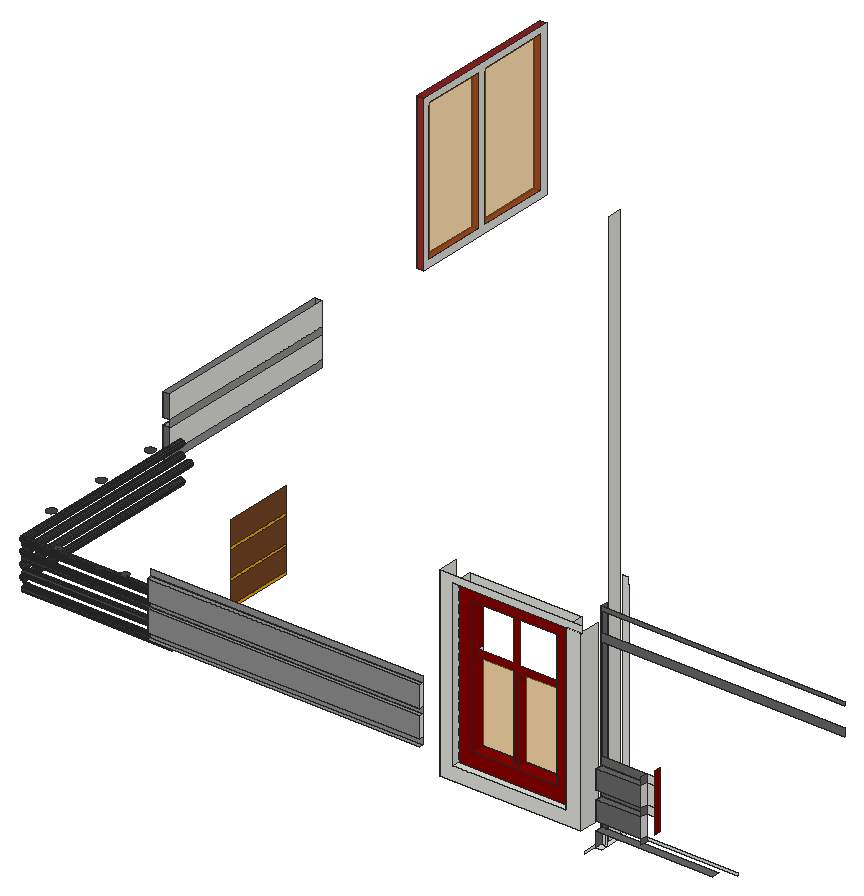
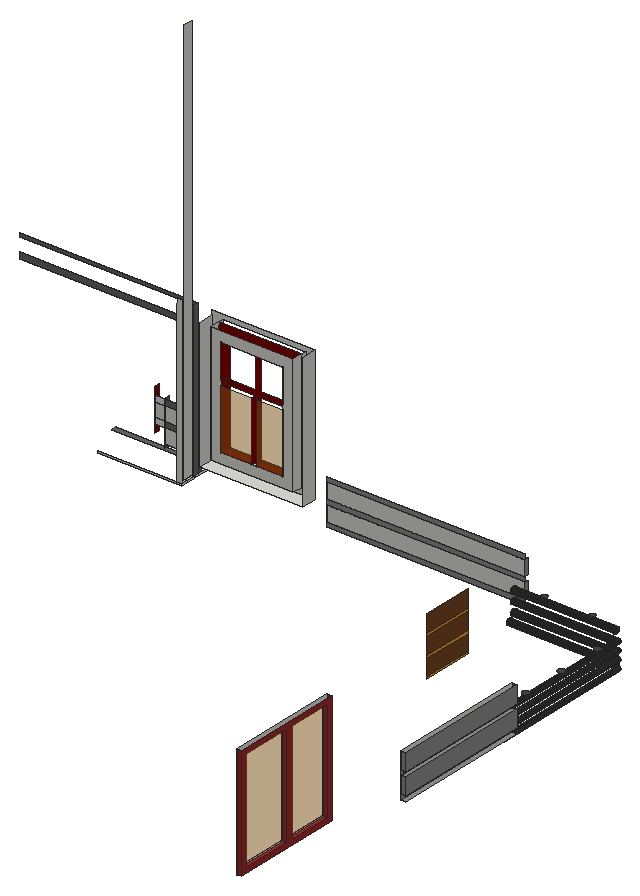
# SketchUp Ruby script. Lengths in inches.
U = 1.inch
M = Sketchup.active_model
def pt(a) = Geom::Point3d.new(a.map { |v| v * U })
def face(e, loops, mat)
  f = e.add_face(loops[0].map { |a| pt(a) })
  loops[1..].each { |l| e.add_face(l.map { |a| pt(a) }).erase! }
  f.material = f.back_material = mat if mat
  f
end
# faces: each face lists its corners as indices into pts; further lists are holes
def faces(e, pts, list, mat = nil) = list.each { |f| face(e, (f[0].is_a?(Array) ? f : [f]).map { |l| l.map { |i| pts[i] } }, mat) }
# xy, xz, yz: faces in a plane at the given z, y or x. An outline is a flat list of corners, or four numbers for a rectangle; further outlines are holes
def ring(l) = l.size == 4 ? [[l[0], l[1]], [l[2], l[1]], [l[2], l[3]], [l[0], l[3]]] : l.each_slice(2).to_a
def flat(e, list, mat, &to3) = list.each { |f| face(e, (f[0].is_a?(Array) ? f : [f]).map { |l| ring(l).map { |u, v| to3.(u, v) } }, mat) }
def xy(e, z, list, mat = nil) = flat(e, list, mat) { |x, y| [x, y, z] }
def xz(e, y, list, mat = nil) = flat(e, list, mat) { |x, z| [x, y, z] }
def yz(e, x, list, mat = nil) = flat(e, list, mat) { |y, z| [x, y, z] }
def lines(e, pts, list) = list.each { |a, b| e.add_line(pt(pts[a]), pt(pts[b])) }
# prism: a flat outline (further loops are holes) pulled along v
def prism(e, loops, v, mat = nil)
  f = face(e, loops, mat); d = Geom::Vector3d.new(v.map { |x| x * U })
  f.pushpull(f.normal.samedirection?(d) ? d.length : -d.length)
end
def box(e, o, s, mat = nil) = prism(e, [[o, [o[0] + s[0], o[1], o[2]], [o[0] + s[0], o[1] + s[1], o[2]], [o[0], o[1] + s[1], o[2]]]], [0, 0, s[2]], mat)
def at(x, y, z, deg = 0) = Geom::Transformation.translation(pt([x, y, z])) * Geom::Transformation.rotation(ORIGIN, Z_AXIS, deg.degrees)
def axes(o, x, y, z) = Geom::Transformation.new([*x, 0, *y, 0, *z, 0, *pt(o).to_a, 1])
def part(name) = M.definitions.add(name)
# library, detail: a bought-in or finely detailed component or shape, given as its bounding box
def library(name, o, s) = part(name).tap { |d| box(d.entities, o, s) }
def detail(e, o, s) = box(e.add_group.entities, o, s)
def put(e, d, t, mat = nil) = e.add_instance(d, t).tap { |i| i.material = mat if mat }
def group(e, t, mat = nil) = e.add_group.tap { |g| g.transformation = t; g.material = mat if mat }.entities
root = M.entities
M.materials.add("[0018_Brown]").color = [165, 42, 42]
M.materials.add("[0021_DarkRed]").color = [139, 0, 0]
M.materials.add("[0038_Orange]").color = [255, 165, 0]
M.materials.add("[0134_DimGray]").color = [105, 105, 105]
M.materials.add("[0137_Black]").color = [71, 71, 71]
M.materials.add("[Color M05]").color = [145, 145, 145]
M.materials.add("[Translucent Glass Gray]").color = [191, 123, 24]
M.materials["[Translucent Glass Gray]"].alpha = 0.5
M.materials.add("[Wood Veneer 01]").color = [120, 70, 37]
xy(root,135.98,[[284.66,7.0625,286.99,10.0625],[284.41,10.0625,286.99,22.0625]])
xy(root,137.03,[[284.41,10.0625,284.66,12.1875],[284.41,12.1875,284.66,13.0625],[284.66,12.1875,284.66,13.0625,284.41,13.0625,284.41,18.1875,285.29,18.1875,285.29,12.1875],[285.29,12.1875,286.17,18.1875],[284.41,18.1875,285.29,22.0625],
  [285.29,18.1875,286.17,22.0625]])
xy(root,141.65,[[82.85,16.375,200.79,18.1875]],"[Color M05]")
xy(root,142.03,[[8.875,116.75,11.875,199.5]],"[Color M05]")
xy(root,142.6875,[[284.66,7.0625,335.53,10.0625]],"[0134_DimGray]")
xy(root,142.96,[[219.91,3.1875,281.16,12.1875]])
xy(root,144.55,[[82.85,16.375,200.79,18.1875]])
xy(root,145.07,[[8.875,116.75,11.875,199.5]],"[Color M05]")
xy(root,146.27,[[284.66,7.0625,304.13,10.0625]],"[0134_DimGray]")
xy(root,148.83,[[225.66,3.1875,274.54,6.1875],[225.66,6.1875,274.54,12.1875]])
xy(root,153.65,[[82.85,16.375,200.79,18.1875]],"[Color M05]")
xy(root,154.6875,[[284.66,7.0625,304.13,10.0625]],"[0134_DimGray]")
xy(root,154.6875,[[15.96,45.8,16.47,45.87,16.93,46.06,17.33,46.37,17.64,46.77,17.84,47.24,17.9,47.74,17.84,48.24,17.64,48.71,17.33,49.11,16.93,49.41,16.47,49.61,15.96,49.67,15.46,49.61,15,49.41,14.59,49.11,14.29,48.71,14.09,48.24,14.03,47.74,14.09,47.24,14.29,46.77,14.59,46.37,15,46.06,15.46,45.87],[15.96,72.86,16.47,72.93,16.93,73.12,17.33,73.43,17.64,73.83,17.84,74.3,17.9,74.8,17.84,75.3,17.64,75.77,17.33,76.17,16.93,76.48,16.47,76.67,15.96,76.74,15.46,76.67,15,76.48,14.59,76.17,14.29,75.77,14.09,75.3,14.03,74.8,14.09,74.3,14.29,73.83,14.59,73.43,15,73.12,15.46,72.93]],"[0137_Black]")
xy(root,154.75,[[15.96,99.36,16.47,99.43,16.93,99.62,17.33,99.93,17.64,100.33,17.84,100.8,17.9,101.3,17.84,101.8,17.64,102.27,17.33,102.67,16.93,102.98,16.47,103.17,15.96,103.24,15.46,103.17,15,102.98,14.59,102.67,14.29,102.27,14.09,101.8,14.03,101.3,14.09,100.8,14.29,100.33,14.59,99.93,15,99.62,15.46,99.43]],"[0137_Black]")
xy(root,154.83,[[247.4,9.1875,250.1,12.1875]])
xy(root,154.83,[[231.66,6.1875,268.54,6.1875,268.54,12.1875,250.1,12.1875,250.1,9.1875,247.4,9.1875,247.4,12.1875,231.66,12.1875]],"[0021_DarkRed]")
xy(root,155.15,[[8.875,116.75,11.875,199.5]],"[Color M05]")
xy(root,155.78,[[8.875,254.47,11.875,321.35]],"[0018_Brown]")
xy(root,156.3125,[[35.53,25.16,35.9375,25.1875,36.32,25.32,36.66,25.54,36.93,25.85,37.11,26.21,37.2,26.61,37.17,27.02,37.04,27.41,36.82,27.75,36.51,28.02,36.15,28.2,35.75,28.28,35.34,28.25,34.95,28.125,34.61,27.9,34.34,27.59,34.16,27.23,34.08,26.83,34.1,26.42,34.23,26.04,34.46,25.7,34.76,25.43,35.13,25.24],[64.53,25.16,64.9375,25.1875,65.32,25.32,65.66,25.54,65.93,25.85,66.11,26.21,66.2,26.61,66.17,27.02,66.04,27.41,65.82,27.75,65.51,28.02,65.15,28.2,64.75,28.28,64.34,28.25,63.95,28.125,63.61,27.9,63.34,27.59,63.16,27.23,63.08,26.83,63.1,26.42,63.23,26.04,63.46,25.7,63.76,25.43,64.13,25.24]],"[0137_Black]")
xy(root,156.55,[[82.85,16.375,200.79,18.1875]])
xy(root,158.19,[[8.875,116.75,11.875,199.5]],"[Color M05]")
xy(root,158.27,[[284.66,7.0625,304.13,10.0625]],"[0134_DimGray]")
xy(root,158.78,[[8.875,257.47,11.875,284.27],[8.875,287.91,11.875,318.35]],"[0018_Brown]")
xy(root,165.65,[[82.85,16.375,200.79,18.1875]],"[Color M05]")
xy(root,166.6875,[[284.66,7.0625,304.13,10.0625]],"[0134_DimGray]")
xz(root,3.1875,[[219.91,142.96,281.16,142.96,281.16,219.83,274.54,219.83,274.54,148.83,225.66,148.83,225.66,219.83,281.47,219.83,281.47,222.71,219.91,222.71]])
xz(root,6.1875,[[[225.66,148.83,274.54,219.83],[231.66,154.83,268.54,213.83]]],"[0021_DarkRed]")
xz(root,7.0625,[[284.66,146.27,304.13,154.6875],[284.66,158.27,304.13,166.6875]],"[0134_DimGray]")
xz(root,9.1875,[[247.4,154.83,250.1,154.83,250.1,190.54,268.54,190.54,268.54,193.6,250.1,193.6,250.1,213.83,247.4,213.83,247.4,193.6,231.66,193.6,231.66,190.54,247.4,190.54]],"[0021_DarkRed]")
xz(root,10.0625,[[284.41,135.98,284.66,137.03],[284.66,135.98,286.17,142.6875],[286.17,135.98,286.99,142.6875],[284.66,146.27,286.17,154.6875],[286.17,146.27,286.99,154.6875],
  [286.99,146.27,304.13,154.6875],[304.13,154.6875,310.13,158.27],[284.66,158.27,286.17,166.6875],[286.17,158.27,286.99,166.6875],[286.99,158.27,304.13,166.6875],
  [304.13,158.27,310.13,166.6875],[304.13,166.6875,310.13,170.27]])
xz(root,10.0625,[[284.41,137.03,284.66,137.03,284.66,214.6875,390.0625,214.6875,390.0625,218.27,284.66,218.27,284.66,226.6875,390.0625,226.6875,390.0625,228.47,284.41,228.47],[284.66,154.6875,304.13,158.27],[284.66,166.6875,304.13,170.27]],"[0134_DimGray]")
xz(root,12.1875,[[[225.66,148.83,274.54,219.83],[231.66,154.83,268.54,213.83]]])
xz(root,12.1875,[[231.66,154.83,247.4,190.54],[250.1,154.83,268.54,190.54]],"[Translucent Glass Gray]")
xz(root,13.0625,[[284.41,137.03,284.66,228.47]])
xz(root,16.375,[[82.85,144.55,200.79,153.65],[82.85,156.55,200.79,165.65]],"[Color M05]")
xz(root,18.1875,[[82.85,144.55,200.79,153.65],[82.85,156.55,200.79,165.65]])
xz(root,18.1875,[[82.85,141.65,200.79,144.55],[82.85,153.65,200.79,156.55],[82.85,165.65,200.79,168.55]],"[Color M05]")
xz(root,22.0625,[[284.41,135.98,286.99,137.03],[286.99,135.98,334.1,137.03],[284.41,137.03,286.99,137.03,286.99,232.22,286.52,232.22,286.52,235.42,284.41,235.42]])
xz(root,116.75,[[8.875,145.07,11.875,155.15],[8.875,158.19,11.875,168.28]],"[0134_DimGray]")
xz(root,121.3125,[[17.02,139.87,16.66,139.91,16.33,140.05,16.05,140.27,15.83,140.55,15.69,140.89,15.65,141.24,15.69,141.6,15.83,141.93,16.05,142.21,16.33,142.43,16.66,142.57,17.02,142.62,17.375,142.57,17.71,142.43,17.99,142.21,18.21,141.93,18.35,141.6,18.4,141.24,18.35,140.89,18.21,140.55,17.99,140.27,17.71,140.05,17.375,139.91]])
xz(root,199.5,[[8.875,145.07,11.875,155.15],[8.875,158.19,11.875,168.28]],"[Color M05]")
xz(root,254.47,[[8.875,155.78,11.875,222.65]],"[0018_Brown]")
xz(root,257.47,[[8.875,158.78,11.875,219.65]],"[0018_Brown]")
xz(root,284.27,[[8.875,158.78,11.875,219.65]],"[0018_Brown]")
xz(root,287.91,[[8.875,158.78,11.875,219.65]],"[0018_Brown]")
xz(root,318.35,[[8.875,158.78,11.875,219.65]],"[0018_Brown]")
xz(root,321.35,[[8.875,155.78,11.875,222.65]],"[0018_Brown]")
yz(root,8.875,[[[254.47,155.78,321.35,222.65],[287.91,158.78,318.35,219.65],[257.47,158.78,284.27,219.65]]],"[0018_Brown]")
yz(root,8.875,[[116.75,145.07,199.5,155.15],[116.75,158.19,199.5,168.28]],"[Color M05]")
yz(root,11.875,[[116.75,145.07,199.5,155.15],[[254.47,155.78,321.35,222.65],[287.91,158.78,318.35,219.65],[257.47,158.78,284.27,219.65]],[116.75,158.19,199.5,168.28]])
yz(root,11.875,[[116.75,142.03,199.5,145.07],[116.75,155.15,199.5,158.19]],"[Color M05]")
yz(root,11.875,[[257.47,158.78,284.27,219.65],[287.91,158.78,318.35,219.65]],"[Translucent Glass Gray]")
yz(root,82.85,[[61.11,134.05,91.11,135.3],[61.11,145.05,91.11,146.3],[61.11,156.99,91.11,158.23]],"[0038_Orange]")
yz(root,82.85,[[16.375,144.55,18.1875,153.65],[16.375,156.55,18.1875,165.65]],"[Color M05]")
yz(root,82.85,[[61.11,135.3,91.11,145.05],[61.11,146.3,91.11,156.99],[61.11,158.23,91.11,168.92]],"[Wood Veneer 01]")
yz(root,85.375,[[27.125,133.9375,27.5625,133.99,27.97,134.16,28.32,134.43,28.59,134.78,28.75,135.1875,28.8125,135.625,28.75,136.06,28.59,136.47,28.32,136.82,27.97,137.08,27.5625,137.25,27.125,137.3125,26.6875,137.25,26.28,137.08,25.93,136.82,25.66,136.47,25.49,136.06,25.4375,135.625,25.49,135.1875,25.66,134.78,25.93,134.43,26.28,134.16,26.6875,133.99]])
yz(root,200.79,[[16.375,144.55,18.1875,153.65],[16.375,156.55,18.1875,165.65]])
yz(root,219.91,[[3.1875,142.96,12.1875,222.71]])
yz(root,225.66,[[3.1875,148.83,6.1875,219.83],[6.1875,148.83,12.1875,219.83]])
yz(root,231.66,[[6.1875,154.83,12.1875,154.83,12.1875,190.54,9.1875,190.54,9.1875,193.6,12.1875,193.6,12.1875,213.83,6.1875,213.83]],"[0021_DarkRed]")
yz(root,247.4,[[9.1875,154.83,12.1875,190.54]],"[0021_DarkRed]")
yz(root,250.1,[[9.1875,154.83,12.1875,190.54]],"[0021_DarkRed]")
yz(root,268.54,[[6.1875,154.83,6.1875,213.83,12.1875,213.83,12.1875,193.6,9.1875,193.6,9.1875,190.54,12.1875,190.54,12.1875,154.83]],"[0021_DarkRed]")
yz(root,274.54,[[3.1875,148.83,6.1875,219.83],[6.1875,148.83,12.1875,219.83]])
yz(root,281.16,[[3.1875,142.96,12.1875,219.83]])
yz(root,284.41,[[1.0625,135.98,10.0625,137.03],[10.0625,135.98,12.1875,137.03],[12.1875,135.98,13.0625,137.03],[13.0625,135.98,18.1875,137.03],[18.1875,135.98,22.0625,137.03]])
yz(root,284.41,[[10.0625,137.03,13.0625,228.47]],"[0134_DimGray]")
yz(root,284.66,[[7.0625,135.98,10.0625,142.6875],[7.0625,146.27,10.0625,154.6875],[7.0625,158.27,10.0625,166.6875]],"[0134_DimGray]")
yz(root,286.17,[[12.1875,137.03,18.1875,379.43]])
yz(root,304.13,[[7.0625,146.27,10.0625,154.6875],[7.0625,158.27,10.0625,166.6875]])
yz(root,304.13,[[7.0625,143.85,10.0625,146.27],[7.0625,154.6875,10.0625,158.27],[7.0625,166.6875,10.0625,170.27]],"[0134_DimGray]")
yz(root,310.13,[[7.0625,149.85,10.0625,174.59]],"[0021_DarkRed]")
p = [[20.875,26.6875,133.99],[20.875,27.125,133.9375],[85.375,27.125,133.9375],[85.375,26.6875,133.99],[20.875,27.5625,133.99],[85.375,27.5625,133.99],
  [20.875,26.28,134.16],[85.375,26.28,134.16],[20.875,27.97,134.16],[85.375,27.97,134.16],[20.875,25.93,134.43],[85.375,25.93,134.43],
  [20.875,28.32,134.43],[85.375,28.32,134.43],[20.875,25.66,134.78],[85.375,25.66,134.78],[20.875,28.59,134.78],[85.375,28.59,134.78],
  [20.875,25.49,135.1875],[85.375,25.49,135.1875],[20.875,28.75,135.1875],[85.375,28.75,135.1875],[17.02,31.0625,134.93],[16.66,31.0625,134.98],
  [16.66,116.75,134.98],[17.02,116.75,134.93],[17.375,31.0625,134.98],[17.375,116.75,134.98],[16.33,31.0625,135.11],[16.33,116.75,135.11],
  [17.71,31.0625,135.11],[17.71,116.75,135.11],[16.05,31.0625,135.33],[16.05,116.75,135.33],[17.99,31.0625,135.33],[17.99,116.75,135.33],
  [20.875,25.4375,135.625],[85.375,25.4375,135.625],[20.875,28.8125,135.625],[85.375,28.8125,135.625],[15.83,31.0625,135.62],[15.83,116.75,135.62],
  [18.21,31.0625,135.62],[18.21,116.75,135.62],[20.875,25.49,136.06],[85.375,25.49,136.06],[20.875,28.75,136.06],[85.375,28.75,136.06],
  [15.69,31.0625,135.95],[15.69,116.75,135.95],[18.35,31.0625,135.95],[18.35,116.75,135.95],[15.65,31.0625,136.3],[15.65,116.75,136.3],
  [18.4,31.0625,136.3],[18.4,116.75,136.3],[20.875,25.66,136.47],[85.375,25.66,136.47],[20.875,28.59,136.47],[85.375,28.59,136.47],
  [15.69,31.0625,136.66],[15.69,116.75,136.66],[18.35,31.0625,136.66],[18.35,116.75,136.66],[20.875,25.93,136.82],[85.375,25.93,136.82],
  [20.875,28.32,136.82],[85.375,28.32,136.82],[15.83,31.0625,136.99],[15.83,116.75,136.99],[18.21,31.0625,136.99],[18.21,116.75,136.99],
  [20.875,26.28,137.08],[85.375,26.28,137.08],[20.875,27.97,137.08],[85.375,27.97,137.08],[16.05,31.0625,137.28],[16.05,116.75,137.28],
  [17.99,31.0625,137.28],[17.99,116.75,137.28],[20.875,26.6875,137.25],[85.375,26.6875,137.25],[20.875,27.5625,137.25],[85.375,27.5625,137.25],
  [20.875,27.125,137.3125],[85.375,27.125,137.3125],[16.33,31.0625,137.49],[16.33,116.75,137.49],[17.71,31.0625,137.49],[17.71,116.75,137.49],
  [16.66,31.0625,137.63],[16.66,116.75,137.63],[17.375,31.0625,137.63],[17.375,116.75,137.63],[17.02,31.0625,137.68],[17.02,116.75,137.68],
  [20.875,26.6875,139.99],[20.875,27.125,139.9375],[82.85,27.125,139.9375],[82.85,26.6875,139.99],[20.875,27.5625,139.99],[82.85,27.5625,139.99],
  [16.66,31.0625,139.91],[16.33,31.0625,140.05],[16.33,121.3125,140.05],[16.66,121.3125,139.91],[17.02,31.0625,139.87],[17.02,121.3125,139.87],
  [17.375,31.0625,139.91],[17.375,121.3125,139.91],[17.71,31.0625,140.05],[17.71,121.3125,140.05],[20.875,26.28,140.16],[82.85,26.28,140.16],
  [20.875,27.97,140.16],[82.85,27.97,140.16],[16.05,31.0625,140.27],[16.05,121.3125,140.27],[17.99,31.0625,140.27],[17.99,121.3125,140.27],
  [20.875,25.93,140.43],[82.85,25.93,140.43],[20.875,28.32,140.43],[82.85,28.32,140.43],[15.83,31.0625,140.55],[15.83,121.3125,140.55],
  [18.21,31.0625,140.55],[18.21,121.3125,140.55],[20.875,25.66,140.78],[82.85,25.66,140.78],[20.875,28.59,140.78],[82.85,28.59,140.78],
  [15.69,31.0625,140.89],[15.69,121.3125,140.89],[18.35,31.0625,140.89],[18.35,121.3125,140.89],[20.875,25.49,141.1875],[82.85,25.49,141.1875],
  [20.875,28.75,141.1875],[82.85,28.75,141.1875],[15.65,31.0625,141.24],[15.65,121.3125,141.24],[18.4,31.0625,141.24],[18.4,121.3125,141.24],
  [20.875,25.4375,141.625],[82.85,25.4375,141.625],[20.875,28.8125,141.625],[82.85,28.8125,141.625],[15.69,31.0625,141.6],[15.69,121.3125,141.6],
  [18.35,31.0625,141.6],[18.35,121.3125,141.6],[20.875,25.49,142.06],[82.85,25.49,142.06],[20.875,28.75,142.06],[82.85,28.75,142.06],
  [15.83,31.0625,141.93],[15.83,121.3125,141.93],[18.21,31.0625,141.93],[18.21,121.3125,141.93],[16.05,31.0625,142.21],[16.05,121.3125,142.21],
  [17.99,31.0625,142.21],[17.99,121.3125,142.21],[20.875,25.66,142.47],[82.85,25.66,142.47],[20.875,28.59,142.47],[82.85,28.59,142.47],
  [16.33,31.0625,142.43],[16.33,121.3125,142.43],[17.71,31.0625,142.43],[17.71,121.3125,142.43],[16.66,31.0625,142.57],[16.66,121.3125,142.57],
  [17.375,31.0625,142.57],[17.375,121.3125,142.57],[20.875,25.93,142.82],[82.85,25.93,142.82],[20.875,28.32,142.82],[82.85,28.32,142.82],
  [17.02,31.0625,142.62],[17.02,121.3125,142.62],[20.875,26.28,143.08],[82.85,26.28,143.08],[20.875,27.97,143.08],[82.85,27.97,143.08],
  [20.875,26.6875,143.25],[82.85,26.6875,143.25],[20.875,27.5625,143.25],[82.85,27.5625,143.25],[20.875,27.125,143.3125],[82.85,27.125,143.3125],
  [17.02,31.0625,144.8],[16.66,31.0625,144.85],[16.66,116.75,144.85],[17.02,116.75,144.8],[17.375,31.0625,144.85],[17.375,116.75,144.85],
  [16.33,31.0625,144.99],[16.33,116.75,144.99],[17.71,31.0625,144.99],[17.71,116.75,144.99],[16.05,31.0625,145.21],[16.05,116.75,145.21],
  [17.99,31.0625,145.21],[17.99,116.75,145.21],[15.83,31.0625,145.49],[15.83,116.75,145.49],[18.21,31.0625,145.49],[18.21,116.75,145.49],
  [15.69,31.0625,145.82],[15.69,116.75,145.82],[18.35,31.0625,145.82],[18.35,116.75,145.82],[15.65,31.0625,146.18],[15.65,116.75,146.18],
  [18.4,31.0625,146.18],[18.4,116.75,146.18],[20.875,26.6875,145.99],[20.875,27.125,145.9375],[82.85,27.125,145.9375],[82.85,26.6875,145.99],
  [20.875,27.5625,145.99],[82.85,27.5625,145.99],[20.875,26.28,146.16],[82.85,26.28,146.16],[20.875,27.97,146.16],[82.85,27.97,146.16],
  [20.875,25.93,146.43],[82.85,25.93,146.43],[20.875,28.32,146.43],[82.85,28.32,146.43],[15.69,31.0625,146.54],[15.69,116.75,146.54],
  [18.35,31.0625,146.54],[18.35,116.75,146.54],[20.875,25.66,146.78],[82.85,25.66,146.78],[20.875,28.59,146.78],[82.85,28.59,146.78],
  [15.83,31.0625,146.87],[15.83,116.75,146.87],[18.21,31.0625,146.87],[18.21,116.75,146.87],[20.875,25.49,147.1875],[82.85,25.49,147.1875],
  [20.875,28.75,147.1875],[82.85,28.75,147.1875],[16.05,31.0625,147.15],[16.05,116.75,147.15],[17.99,31.0625,147.15],[17.99,116.75,147.15],
  [20.875,25.4375,147.625],[82.85,25.4375,147.625],[20.875,28.8125,147.625],[82.85,28.8125,147.625],[16.33,31.0625,147.37],[16.33,116.75,147.37],
  [17.71,31.0625,147.37],[17.71,116.75,147.37],[16.66,31.0625,147.51],[16.66,116.75,147.51],[17.375,31.0625,147.51],[17.375,116.75,147.51],
  [17.02,31.0625,147.55],[17.02,116.75,147.55],[20.875,25.49,148.06],[82.85,25.49,148.06],[20.875,28.75,148.06],[82.85,28.75,148.06],
  [20.875,25.66,148.47],[82.85,25.66,148.47],[20.875,28.59,148.47],[82.85,28.59,148.47],[20.875,25.93,148.82],[82.85,25.93,148.82],
  [20.875,28.32,148.82],[82.85,28.32,148.82],[20.875,26.28,149.08],[82.85,26.28,149.08],[20.875,27.97,149.08],[82.85,27.97,149.08],
  [20.875,26.6875,149.25],[82.85,26.6875,149.25],[20.875,27.5625,149.25],[82.85,27.5625,149.25],[20.875,27.125,149.3125],[82.85,27.125,149.3125],
  [17.02,31.0625,149.74],[16.66,31.0625,149.79],[16.66,116.75,149.79],[17.02,116.75,149.74],[17.375,31.0625,149.79],[17.375,116.75,149.79],
  [16.33,31.0625,149.93],[16.33,116.75,149.93],[17.71,31.0625,149.93],[17.71,116.75,149.93],[16.05,31.0625,150.14],[16.05,116.75,150.14],
  [17.99,31.0625,150.14],[17.99,116.75,150.14],[15.83,31.0625,150.43],[15.83,116.75,150.43],[18.21,31.0625,150.43],[18.21,116.75,150.43],
  [15.69,31.0625,150.76],[15.69,116.75,150.76],[18.35,31.0625,150.76],[18.35,116.75,150.76],[15.65,31.0625,151.12],[15.65,116.75,151.12],
  [18.4,31.0625,151.12],[18.4,116.75,151.12],[15.69,31.0625,151.47],[15.69,116.75,151.47],[18.35,31.0625,151.47],[18.35,116.75,151.47],
  [15.83,31.0625,151.8],[15.83,116.75,151.8],[18.21,31.0625,151.8],[18.21,116.75,151.8],[16.05,31.0625,152.09],[16.05,116.75,152.09],
  [17.99,31.0625,152.09],[17.99,116.75,152.09],[20.875,26.6875,151.99],[20.875,27.125,151.9375],[82.85,27.125,151.9375],[82.85,26.6875,151.99],
  [20.875,27.5625,151.99],[82.85,27.5625,151.99],[20.875,26.28,152.16],[82.85,26.28,152.16],[20.875,27.97,152.16],[82.85,27.97,152.16],
  [16.33,31.0625,152.31],[16.33,116.75,152.31],[17.71,31.0625,152.31],[17.71,116.75,152.31],[20.875,25.93,152.43],[82.85,25.93,152.43],
  [20.875,28.32,152.43],[82.85,28.32,152.43],[16.66,31.0625,152.44],[16.66,116.75,152.44],[17.375,31.0625,152.44],[17.375,116.75,152.44],
  [20.875,25.66,152.78],[82.85,25.66,152.78],[20.875,28.59,152.78],[82.85,28.59,152.78],[17.02,31.0625,152.49],[17.02,116.75,152.49],
  [20.875,25.49,153.1875],[82.85,25.49,153.1875],[20.875,28.75,153.1875],[82.85,28.75,153.1875],[20.875,25.4375,153.625],[82.85,25.4375,153.625],
  [20.875,28.8125,153.625],[82.85,28.8125,153.625],[20.875,25.49,154.06],[82.85,25.49,154.06],[20.875,28.75,154.06],[82.85,28.75,154.06],
  [20.875,25.66,154.47],[82.85,25.66,154.47],[20.875,28.59,154.47],[82.85,28.59,154.47],[20.875,25.93,154.82],[82.85,25.93,154.82],
  [20.875,28.32,154.82],[82.85,28.32,154.82],[20.875,26.28,155.08],[82.85,26.28,155.08],[20.875,27.97,155.08],[82.85,27.97,155.08],
  [20.875,26.6875,155.25],[82.85,26.6875,155.25],[20.875,27.5625,155.25],[82.85,27.5625,155.25],[20.875,27.125,155.3125],[82.85,27.125,155.3125]]
faces(root,p,[[0,1,2,3],[1,4,5,2],[6,0,3,7],[4,8,9,5],[10,6,7,11],[8,12,13,9],[14,10,11,15],[12,16,17,13],
  [18,14,15,19],[16,20,21,17],[22,23,24,25],[26,22,25,27],[23,28,29,24],[30,26,27,31],[28,32,33,29],[34,30,31,35],
  [36,18,19,37],[20,38,39,21],[32,40,41,33],[42,34,35,43],[44,36,37,45],[38,46,47,39],[40,48,49,41],[50,42,43,51],
  [48,52,53,49],[54,50,51,55],[56,44,45,57],[46,58,59,47],[52,60,61,53],[62,54,55,63],[64,56,57,65],[58,66,67,59],
  [60,68,69,61],[70,62,63,71],[72,64,65,73],[66,74,75,67],[68,76,77,69],[78,70,71,79],[80,72,73,81],[74,82,83,75],
  [84,80,81,85],[82,84,85,83],[76,86,87,77],[88,78,79,89],[86,90,91,87],[92,88,89,93],[90,94,95,91],[94,92,93,95],
  [96,97,98,99],[97,100,101,98],[102,103,104,105],[106,102,105,107],[108,106,107,109],[110,108,109,111],[112,96,99,113],[100,114,115,101],
  [103,116,117,104],[118,110,111,119],[120,112,113,121],[114,122,123,115],[116,124,125,117],[126,118,119,127],[128,120,121,129],[122,130,131,123],
  [124,132,133,125],[134,126,127,135],[136,128,129,137],[130,138,139,131],[132,140,141,133],[142,134,135,143],[144,136,137,145],[138,146,147,139],
  [140,148,149,141],[150,142,143,151],[152,144,145,153],[146,154,155,147],[148,156,157,149],[158,150,151,159],[156,160,161,157],[162,158,159,163],
  [164,152,153,165],[154,166,167,155],[160,168,169,161],[170,162,163,171],[168,172,173,169],[174,170,171,175],[176,164,165,177],[166,178,179,167],
  [172,180,181,173],[180,174,175,181],[182,176,177,183],[178,184,185,179],[186,182,183,187],[184,188,189,185],[190,186,187,191],[188,190,191,189],
  [192,193,194,195],[196,192,195,197],[193,198,199,194],[200,196,197,201],[198,202,203,199],[204,200,201,205],[202,206,207,203],[208,204,205,209],
  [206,210,211,207],[212,208,209,213],[210,214,215,211],[216,212,213,217],[218,219,220,221],[219,222,223,220],[224,218,221,225],[222,226,227,223],
  [228,224,225,229],[226,230,231,227],[214,232,233,215],[234,216,217,235],[236,228,229,237],[230,238,239,231],[232,240,241,233],[242,234,235,243],
  [244,236,237,245],[238,246,247,239],[240,248,249,241],[250,242,243,251],[252,244,245,253],[246,254,255,247],[248,256,257,249],[258,250,251,259],
  [256,260,261,257],[262,258,259,263],[260,264,265,261],[264,262,263,265],[266,252,253,267],[254,268,269,255],[270,266,267,271],[268,272,273,269],
  [274,270,271,275],[272,276,277,273],[278,274,275,279],[276,280,281,277],[282,278,279,283],[280,284,285,281],[286,282,283,287],[284,286,287,285],
  [288,289,290,291],[292,288,291,293],[289,294,295,290],[296,292,293,297],[294,298,299,295],[300,296,297,301],[298,302,303,299],[304,300,301,305],
  [302,306,307,303],[308,304,305,309],[306,310,311,307],[312,308,309,313],[310,314,315,311],[316,312,313,317],[314,318,319,315],[320,316,317,321],
  [318,322,323,319],[324,320,321,325],[326,327,328,329],[327,330,331,328],[332,326,329,333],[330,334,335,331],[322,336,337,323],[338,324,325,339],
  [340,332,333,341],[334,342,343,335],[336,344,345,337],[346,338,339,347],[348,340,341,349],[342,350,351,343],[344,352,353,345],[352,346,347,353],
  [354,348,349,355],[350,356,357,351],[358,354,355,359],[356,360,361,357],[362,358,359,363],[360,364,365,361],[366,362,363,367],[364,368,369,365],
  [370,366,367,371],[368,372,373,369],[374,370,371,375],[372,376,377,373],[378,374,375,379],[376,380,381,377],[382,378,379,383],[380,382,383,381]],"[0137_Black]")
